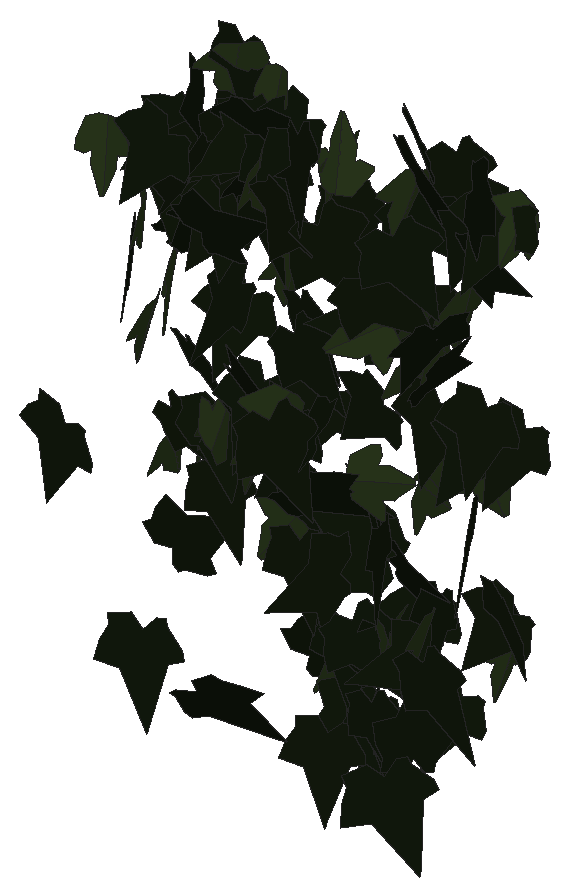
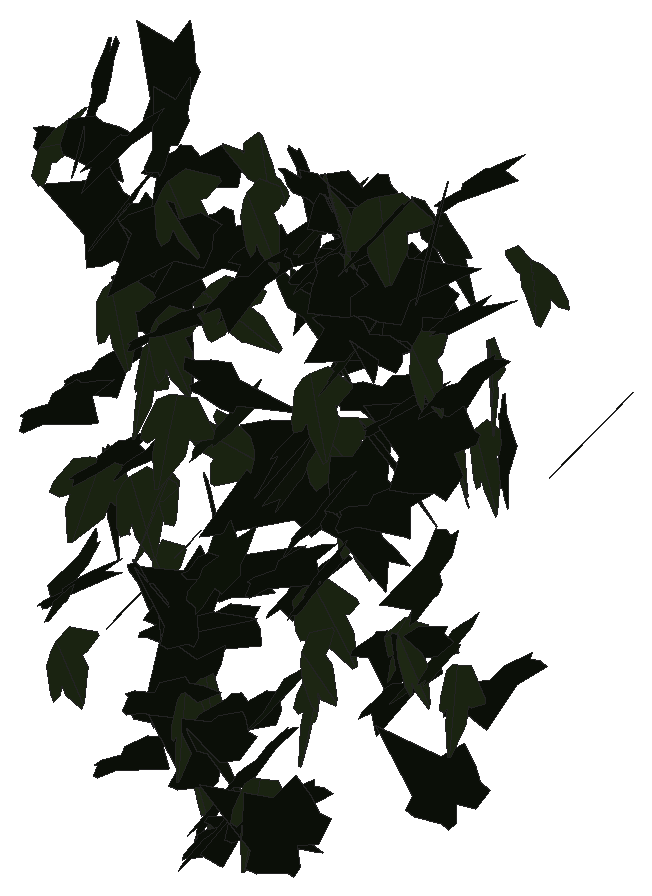
# SketchUp Ruby script. Lengths in inches.
U = 1.inch
M = Sketchup.active_model
def pt(a) = Geom::Point3d.new(a.map { |v| v * U })
def face(e, loops, mat)
  f = e.add_face(loops[0].map { |a| pt(a) })
  loops[1..].each { |l| e.add_face(l.map { |a| pt(a) }).erase! }
  f.material = f.back_material = mat if mat
  f
end
# faces: each face lists its corners as indices into pts; further lists are holes
def faces(e, pts, list, mat = nil) = list.each { |f| face(e, (f[0].is_a?(Array) ? f : [f]).map { |l| l.map { |i| pts[i] } }, mat) }
# xy, xz, yz: faces in a plane at the given z, y or x. An outline is a flat list of corners, or four numbers for a rectangle; further outlines are holes
def ring(l) = l.size == 4 ? [[l[0], l[1]], [l[2], l[1]], [l[2], l[3]], [l[0], l[3]]] : l.each_slice(2).to_a
def flat(e, list, mat, &to3) = list.each { |f| face(e, (f[0].is_a?(Array) ? f : [f]).map { |l| ring(l).map { |u, v| to3.(u, v) } }, mat) }
def xy(e, z, list, mat = nil) = flat(e, list, mat) { |x, y| [x, y, z] }
def xz(e, y, list, mat = nil) = flat(e, list, mat) { |x, z| [x, y, z] }
def yz(e, x, list, mat = nil) = flat(e, list, mat) { |y, z| [x, y, z] }
def lines(e, pts, list) = list.each { |a, b| e.add_line(pt(pts[a]), pt(pts[b])) }
# prism: a flat outline (further loops are holes) pulled along v
def prism(e, loops, v, mat = nil)
  f = face(e, loops, mat); d = Geom::Vector3d.new(v.map { |x| x * U })
  f.pushpull(f.normal.samedirection?(d) ? d.length : -d.length)
end
def box(e, o, s, mat = nil) = prism(e, [[o, [o[0] + s[0], o[1], o[2]], [o[0] + s[0], o[1] + s[1], o[2]], [o[0], o[1] + s[1], o[2]]]], [0, 0, s[2]], mat)
def at(x, y, z, deg = 0) = Geom::Transformation.translation(pt([x, y, z])) * Geom::Transformation.rotation(ORIGIN, Z_AXIS, deg.degrees)
def axes(o, x, y, z) = Geom::Transformation.new([*x, 0, *y, 0, *z, 0, *pt(o).to_a, 1])
def part(name) = M.definitions.add(name)
# library, detail: a bought-in or finely detailed component or shape, given as its bounding box
def library(name, o, s) = part(name).tap { |d| box(d.entities, o, s) }
def detail(e, o, s) = box(e.add_group.entities, o, s)
def put(e, d, t, mat = nil) = e.add_instance(d, t).tap { |i| i.material = mat if mat }
def group(e, t, mat = nil) = e.add_group.tap { |g| g.transformation = t; g.material = mat if mat }.entities
root = M.entities
M.materials.add("efeu1").color = [18, 25, 13]
M.materials.add("efeu2").color = [43, 57, 29]
c1 = part("ivyleaf_9")
p = [[1.54,2.16,1.25],[1.36,2.04,1.19],[-0.21,0.99,0.68],[-0.71,1.11,0.82],[-0.85,0.86,0.67],[-0.8,0.17,0.21],
  [-0.9,-0.01,0.1],[-0.67,-0.16,-0.02],[-0.08,-0.08,-0.05],[-0.03,-0.6,-0.4],[0.65,-0.88,-0.66],[0.83,-0.6,-0.49],
  [1.29,-0.42,-0.43],[1.8125,-0.07,-0.26],[1.21,0.44,0.15]]
faces(c1.entities,p,[[0,1,2,3,4,5,6,7,8,9,10,11,12,13,14]],"efeu1")
c2 = part("ivyleaf_10")
p = [[0,0.5,-0.03],[-0.0625,2.02,-0.43],[-0.19,2.01,-0.46],[-0.54,1.05,-0.29],[-0.52,0.625,-0.18],[-0.83,0.76,-0.28],
  [-1.16,0.64,-0.33],[-1.15,0.33,-0.24],[-0.77,-0.39,0.02],[-0.3,-0.51,0.16],[0.04,-0.48,0.23],[-0.02,2.01,-0.4375],
  [-0.06,2.01,-0.43],[0.04,-0.49,0.23],[0.67,-0.49,0.14],[1.38,0.36,-0.2],[1.375,0.51,-0.24],[0.81,0.65,-0.19],
  [0.62,0.59,-0.15],[0.6,1.09,-0.28],[0.5,1.23,-0.31]]
faces(c2.entities,p,[[0,1,2,3,4,5,6,7,8,9,10],[11,12,0,13,14,15,16,17,18,19,20]],"efeu2")
put(root,c1,axes([577.89,105.38,287.08],[1.36278,0.54862,0.30222],[0.27821,0.11819,-1.46906],[-0.56118,1.39088,0.00562]))
put(root,c1,axes([563.9,114.26,290.22],[-0.08091,-1.18047,0.66258],[0.11331,-0.66733,-1.17511],[1.34895,-0.01475,0.13845]))
put(root,c1,axes([574.375,114.15,293.99],[0.26304,-1.18109,-0.79581],[-0.14529,0.7828,-1.20979],[1.41675,0.29956,0.02369]))
put(root,c1,axes([566.35,116.12,281.01],[-0.09475,-1.31976,-0.20399],[0.02309,0.20285,-1.32313],[1.33524,-0.09716,0.00841]))
put(root,c1,axes([578.76,115.81,278.92],[-0.22824,-1.01787,-0.89838],[0.1809,0.88006,-1.04307],[1.34552,-0.29098,-0.01215]))
put(root,c1,axes([575.25,115.64,293.05],[-0.94436,1.02445,0.23829],[-0.18259,0.15571,-1.39303],[-1.03583,-0.96143,0.0283]))
put(root,c1,axes([575.72,116.52,286.74],[-1.25986,0.4566,0.27428],[-0.252,0.10961,-1.33995],[-0.46927,-1.28471,-0.01684]))
put(root,c1,axes([565.27,118.89,301.64],[-0.52851,-1.00941,0.55527],[-0.07084,-0.58128,-1.12412],[1.14988,-0.49976,0.18595]))
put(root,c1,axes([578.23,118.9375,282.4],[0.70807,-1.23112,-0.31612],[-0.01276,0.35496,-1.41095],[1.27099,0.68942,0.16195]))
put(root,c1,axes([572.15,118.625,288.33],[1.21039,0.63768,0.61607],[0.52332,0.32779,-1.36745],[-0.71576,1.31801,0.04201]))
put(root,c2,axes([569.98,120.21,290.71],[-0.43783,-0.87738,0.74683],[-0.04292,-0.78596,-0.94851],[1.15139,-0.36293,0.24863]))
put(root,c2,axes([561.52,119.76,300.16],[1.20036,-0.19085,0.29262],[0.28978,-0.04099,-1.21543],[0.19514,1.23483,0.00488]))
put(root,c1,axes([571.11,120.01,284.96],[0.15727,-1.22297,-0.12797],[0.00639,0.12983,-1.23283],[1.22963,0.15574,0.02278]))
put(root,c1,axes([566.16,119.18,300.13],[-0.65049,1.03551,0.3217],[-0.19726,0.25588,-1.22251],[-1.06624,-0.67909,0.0299]))
put(root,c1,axes([570.03,120.67,299.14],[-0.21173,-0.90489,0.90272],[0.23072,-0.92705,-0.87516],[1.25718,0.01773,0.31264]))
put(root,c2,axes([577.16,120.29,283.33],[0.4807,-1.10236,0.33779],[0.12234,-0.31513,-1.20254],[1.14644,0.49584,-0.01331]))
put(root,c2,axes([563.58,120.07,292.78],[0.34272,-1.17563,0.02611],[0.00411,-0.026,-1.22456],[1.17591,0.34273,-0.00333]))
put(root,c1,axes([576.95,120.68,281.52],[-0.79447,-0.34135,0.79792],[-0.63668,-0.50589,-0.85035],[0.58977,-1.00595,0.15688]))
put(root,c1,axes([577.22,119.47,277.95],[-0.59743,-0.67037,1.00603],[0.67993,0.74154,0.8979],[-0.9996,0.90506,0.00949]))
put(root,c1,axes([574.73,120.51,286.51],[-0.54702,0.00334,-1.18883],[1.17206,-0.21759,-0.53992],[-0.19905,-1.29043,0.08796]))
put(root,c1,axes([566.18,120.21,297.12],[0.157,-0.2934,1.28344],[1.16543,-0.57029,-0.27293],[0.61243,1.16045,0.19036]))
put(root,c2,axes([574.18,120.09,288.9],[0.25921,-0.06776,-1.21929],[1.20348,-0.19721,0.2668],[-0.2071,-1.23084,0.02437]))
put(root,c1,axes([578.26,119.09,295.24],[0.27353,0.98132,0.76722],[0.21056,0.73777,-1.01872],[-1.22771,0.34517,-0.00378]))
put(root,c1,axes([571.91,120.73,276.32],[-0.22673,-1.19319,-0.1831],[0.02861,0.18094,-1.21453],[1.20682,-0.22846,-0.00561]))
put(root,c2,axes([568.76,120.55,288.57],[0.1236,-1.20506,0.1788],[-0.00327,-0.18005,-1.21119],[1.21825,0.12178,-0.02139]))
put(root,c2,axes([575.41,120.62,276.25],[0.58962,-1.08793,0.02339],[0.01036,-0.02099,-1.23743],[1.08813,0.58971,-0.00089]))
put(root,c1,axes([575.9,121.23,302.59],[0.30446,-0.52323,1.26611],[0.66648,-1.07659,-0.60518],[1.19691,0.73257,0.01492]))
put(root,c1,axes([575.5,120.46,299.88],[-0.04129,-0.87034,-0.91332],[0.14047,0.90496,-0.86872],[1.25376,-0.13005,0.06725]))
put(root,c1,axes([567.95,121.35,289.66],[0.97732,-0.73267,0.40156],[-0.30722,0.25954,1.22125],[-0.77696,-1.02423,0.02221]))
put(root,c2,axes([574.05,121.05,295.14],[0.72605,0.11446,-1.00994],[-1.01361,-0.01047,-0.72987],[-0.07534,1.2438,0.0868]))
put(root,c2,axes([562.6,120.77,296.79],[0.58017,-1.01804,-0.39809],[-0.05093,0.42503,-1.16114],[1.09192,0.56074,0.15736]))
put(root,c2,axes([569.86,121.02,284.99],[-0.93809,-0.08041,0.78306],[-0.74688,-0.29386,-0.92492],[0.24864,-1.1861,0.17606]))
put(root,c1,axes([574.13,120.39,297.6],[0.18492,-0.51713,-1.20247],[0.04793,1.21627,-0.5157],[1.30808,0.02854,0.18889]))
put(root,c1,axes([561.35,121.77,294.41],[-0.17003,-0.1695,-1.27422],[1.18432,-0.52035,-0.08882],[-0.49974,-1.17549,0.22305]))
put(root,c1,axes([569.14,122.0625,289.07],[0.03941,-1.2902,0.50679],[-0.02468,-0.50757,-1.29026],[1.38595,0.02765,-0.03738]))
put(root,c1,axes([573.95,121.61,284.69],[-0.79672,-0.92263,-0.46111],[-0.30433,-0.34644,1.21901],[-0.98552,0.85286,-0.00366]))
put(root,c1,axes([569.55,121.77,301.7],[-0.64683,-0.14753,-1.1372],[1.14315,0.0202,-0.65283],[0.0906,-1.30813,0.11817]))
put(root,c1,axes([576.59,121.74,283.55],[-0.8172,-0.09349,-0.84368],[0.84407,0.03448,-0.8214],[0.08986,-1.17406,0.04306]))
put(root,c1,axes([571.26,121.125,298.59],[0.32352,-0.9443,-1.00575],[-0.11667,1.01061,-0.98639],[1.37464,0.30801,0.15299]))
put(root,c1,axes([573.16,122.51,290.77],[-0.51599,-0.70657,0.92485],[0.10306,-1.03544,-0.73355],[1.1593,-0.22244,0.47686]))
put(root,c2,axes([562.93,122.15,293.5],[0.64905,-0.79377,0.75091],[0.56877,-0.50031,-1.02049],[0.93297,0.85721,0.09973]))
put(root,c1,axes([567.26,122.55,300.82],[-0.82698,-0.61661,0.73916],[-0.44091,-0.6236,-1.0135],[0.85567,-0.91726,0.19214]))
put(root,c2,axes([567.83,121.46,299.97],[0.27421,-1.14773,-0.41918],[0.07985,0.44552,-1.16761],[1.21927,0.22895,0.17074]))
put(root,c2,axes([571.76,121.6,300.89],[1.22195,-0.11879,0.25277],[-0.23605,0.16708,1.21964],[-0.14928,-1.23659,0.14051]))
put(root,c1,axes([578.87,121.18,302.86],[0.53115,-0.29829,-1.28915],[-1.07354,0.71496,-0.60774],[0.77356,1.19702,0.04175]))
put(root,c1,axes([568.79,122.93,286.5625],[-0.3129,-0.66714,1.03647],[-0.18543,-1.0317,-0.72004],[1.21859,-0.32829,0.15657]))
put(root,c1,axes([576.28,121.83,295.47],[-0.13088,1.13232,-0.66665],[0.05253,-0.6649,-1.13966],[-1.31293,-0.13948,0.02086]))
put(root,c1,axes([577.69,122.58,287.45],[-0.60065,0.20524,-1.24958],[1.16112,-0.46265,-0.63412],[-0.50534,-1.30698,0.02824]))
put(root,c1,axes([563.8,122.97,300.64],[-0.04151,-0.17225,1.30547],[-0.05253,-1.30486,-0.17384],[1.31574,-0.05753,0.03424]))
put(root,c1,axes([569.25,122.51,302.11],[-1.19732,-0.19335,-0.15528],[0.1564,0.00537,-1.21267],[0.19244,-1.20733,0.01947]))
put(root,c1,axes([567.32,121.84,302.04],[0.71611,0.6531,-0.8491],[-0.65285,-0.54368,-0.96878],[-0.8493,0.96861,0.02874]))
put(root,c1,axes([567.82,122.6,300.03],[0.25555,-1.32619,-0.01949],[-0.00444,0.019,-1.35059],[1.32633,0.25559,-0.00076]))
put(root,c1,axes([572.13,122.79,276.66],[-1.05614,-0.45578,0.43483],[-0.39983,-0.17091,-1.15029],[0.48677,-1.12929,-0.00141]))
put(root,c1,axes([574,122.54,283.78],[0.49409,-0.48091,1.03658],[0.77627,-0.68748,-0.68896],[0.83855,0.91977,0.02702]))
put(root,c1,axes([567.09,122.66,289.51],[-1.06388,-0.42242,-0.52722],[0.51245,0.13628,-1.14326],[0.44022,-1.1795,0.05673]))
put(root,c1,axes([579.05,123.19,283.18],[-0.57956,-0.86263,0.60045],[-0.06256,-0.65616,-1.00304],[1.04916,-0.51564,0.27188]))
put(root,c1,axes([569.26,122.11,292.65],[0.61896,-0.95162,-0.6698],[-0.22478,0.64659,-1.12638],[1.14179,0.64317,0.14135]))
put(root,c1,axes([572.67,122.59,277.15],[0.39567,-1.07385,-0.1602],[-0.0226,0.16232,-1.14391],[1.0855,0.3948,0.03458]))
put(root,c1,axes([577.96,123.04,291.99],[-0.32568,-1.20389,0.10958],[-0.00008,-0.11346,-1.24681],[1.20886,-0.32435,0.02944]))
put(root,c2,axes([573.96,122.01,280.39],[-0.86404,0.37667,0.68619],[-0.65681,0.20714,-0.94075],[-0.42584,-1.08376,0.05869]))
put(root,c1,axes([562.76,123.39,299.03],[-0.68353,-0.64737,0.81932],[-0.28756,-0.82468,-0.89151],[1.00384,-0.67705,0.3025]))
put(root,c1,axes([572.6,122.84,276.11],[-0.09063,-1.14355,-0.11002],[-0.01146,0.11126,-1.14696],[1.14877,-0.08911,-0.02012]))
put(root,c1,axes([572.07,122.21,280.78],[0.1626,-0.85196,-0.84036],[0.04388,0.85176,-0.85502],[1.19587,0.08459,0.14563]))
put(root,c1,axes([572.43,123.39,285.82],[-0.23204,-0.6704,1.11977],[0.42225,-1.11472,-0.57988],[1.23492,0.25519,0.40868]))
put(root,c1,axes([578.73,123.09,283.71],[0.53554,-1.02212,0.40608],[0.15559,-0.37671,-1.15339],[1.08877,0.55659,-0.03491]))
put(root,c1,axes([565.77,122.9,293.35],[-1.23523,0.22734,-0.40711],[0.39898,-0.08129,-1.25595],[-0.24132,-1.29805,0.00736]))
put(root,c1,axes([570.83,123.17,279.5],[0.18261,-1.20725,0.10411],[0.01842,-0.10251,-1.22098],[1.21159,0.18352,0.00287]))
put(root,c1,axes([564.71,122.93,284.45],[0.18753,-1.14588,-0.32734],[0.00398,0.33197,-1.15981],[1.19172,0.17921,0.05539]))
put(root,c1,axes([565.46,123.5625,299.9375],[-0.31332,-0.64155,-1.03911],[-0.12434,-1.05043,0.68603],[-1.21485,0.27296,0.19778]))
put(root,c1,axes([578.79,123.36,301.08],[-0.98853,-0.81503,-0.06027],[0.04514,0.04,-1.28119],[0.81601,-0.98955,-0.00215]))
put(root,c1,axes([567.14,122.53,299.29],[-0.08221,1.21274,-0.3604],[0.01764,-0.36002,-1.21551],[-1.26504,-0.08383,0.00648]))
put(root,c1,axes([573.74,122.81,279.9],[-0.85773,0.78078,-0.06225],[0.03978,-0.04876,-1.15984],[-0.78225,-0.8586,0.00927]))
put(root,c1,axes([562.63,122.84,280.66],[-0.07925,0.05703,1.23905],[1.14165,-0.48202,0.09521],[0.4849,1.14419,-0.02165]))
put(root,c1,axes([569.27,123.75,282.75],[0.05959,-1.11553,0.60498],[0.20415,-0.58933,-1.10679],[1.25249,0.14914,0.15162]))
put(root,c1,axes([574.15,123.73,302.42],[0.23642,-0.65477,1.04571],[0.39283,-0.96938,-0.69579],[1.16958,0.45794,0.02231]))
put(root,c1,axes([576.07,123.74,278.11],[-0.55613,-0.98352,0.2666],[-0.0364,-0.28436,-1.12494],[1.01836,-0.54726,0.10538]))
put(root,c2,axes([575.3,122.39,287.94],[0.35288,-0.86341,-0.86324],[0.21265,0.9283,-0.84156],[1.20226,0.08923,0.40222]))
put(root,c2,axes([574.58,123.39,294.68],[0.17718,-1.18072,0.34133],[0.02181,-0.34179,-1.19362],[1.22888,0.1763,-0.02803]))
put(root,c1,axes([562.56,122.82,286.68],[0.87331,-0.76684,-0.3514],[-0.0934,0.41478,-1.13728],[0.83833,0.84504,0.23935]))
put(root,c1,axes([566.3125,123.54,297.08],[0.5217,-1.14333,0.15498],[0.0618,-0.14215,-1.25673],[1.15213,0.52534,-0.00276]))
put(root,c1,axes([562.96,123.29,289.51],[0.92191,-0.84276,0.21842],[0.15633,-0.1527,-1.24904],[0.85645,0.93504,-0.00712]))
put(root,c2,axes([570.63,123.47,300.98],[0.26889,-1.18359,0.29569],[0.05014,-0.29181,-1.21366],[1.21894,0.2731,-0.01531]))
put(root,c1,axes([572.27,123.64,276.42],[0.2318,-1.16401,0.1185],[0.02964,-0.11492,-1.18685],[1.16965,0.2336,0.00659]))
put(root,c2,axes([579.04,124.05,300.61],[-0.39437,-0.50394,1.0881],[0.54717,-1.09486,-0.30875],[1.06701,0.37519,0.5605]))
put(root,c1,axes([561.63,123.72,297.52],[-0.0306,-1.24024,-0.05442],[0.00363,0.05435,-1.24062],[1.24143,-0.03073,0.00229]))
put(root,c1,axes([576.87,123.29,298.37],[0.60096,0.01997,-1.10127],[1.04017,0.40232,0.57492],[0.36226,-1.18831,0.17613]))
put(root,c2,axes([562.28,122.99,285.36],[0.08574,-1.08727,-0.50464],[0.02221,0.50728,-1.08919],[1.19847,0.06838,0.05628]))
put(root,c2,axes([573.82,123.73,300.41],[-0.13628,-1.16164,0.45441],[0.07742,-0.46411,-1.16321],[1.24495,-0.0983,0.12208]))
put(root,c1,axes([574.73,124.12,290.56],[-0.17607,-1.20745,0.37751],[0.05421,-0.388,-1.21571],[1.26392,-0.15156,0.10473]))
put(root,c2,axes([567.02,123.59,302.6],[1.04102,-0.56831,0.28773],[0.24019,-0.16037,-1.18579],[0.58998,1.06808,-0.02495]))
put(root,c1,axes([578.86,124.18,290.87],[-0.53124,-1.08065,0.28391],[-0.10299,-0.26567,-1.20392],[1.11256,-0.54059,0.02412]))
put(root,c1,axes([564.0625,124.31,295.73],[-0.50955,-0.97476,0.52143],[-0.0376,-0.55854,-1.08088],[1.10482,-0.46858,0.2037]))
put(root,c1,axes([575.98,124.34,299.2],[0.00271,-1.0552,0.65451],[0.02732,-0.6543,-1.05497],[1.2414,0.01671,0.02179]))
put(root,c1,axes([572.6,123.72,293.73],[-0.88933,0.12566,0.81012],[-0.81109,0.03894,-0.89644],[-0.11921,-1.20237,0.05563]))
put(root,c2,axes([564.76,122.5625,286.34],[0.15334,0.52626,-1.12057],[-0.11136,1.13041,0.51564],[1.23297,0.03665,0.18593]))
put(root,c1,axes([574.08,124.41,295.53],[-0.52362,-1.02596,0.45091],[0.02708,-0.50914,-1.12701],[1.12035,-0.4672,0.23799]))
put(root,c2,axes([568.43,123.11,282.95],[-0.92891,0.77239,0.36964],[-0.27685,0.24518,-1.20803],[-0.8103,-0.96923,-0.01101]))
put(root,c2,axes([563.73,123.92,286.61],[0.48002,-1.0968,0.32795],[0.09795,-0.31496,-1.19672],[1.14058,0.48864,-0.03524]))
put(root,c1,axes([564.03,123.78,286.82],[-0.34826,-1.04427,-0.57352],[0.26951,0.51298,-1.09769],[1.16052,-0.43251,0.08282]))
put(root,c1,axes([576.55,124.5,289.59],[-0.5061,-0.9947,0.53894],[-0.10536,-0.5464,-1.10741],[1.12641,-0.49803,0.13856]))
put(root,c1,axes([570.57,123.86,298.53],[0.13608,-1.1957,-0.33329],[-0.05078,0.32964,-1.20335],[1.24024,0.14469,-0.01271]))
put(root,c2,axes([578.42,124.08,281.27],[0.05087,-1.07595,0.45158],[0.17304,-0.44006,-1.06799],[1.15397,0.11342,0.14024]))
put(root,c1,axes([564.98,124.32,291.875],[-0.59813,-1.04604,0.07859],[-0.02907,-0.0739,-1.20492],[1.04859,-0.59872,0.01143]))
put(root,c1,axes([562.42,123.27,294.42],[0.80537,0.85603,-0.56737],[0.39586,0.40655,1.1753],[0.94762,-0.89736,-0.00877]))
put(root,c1,axes([572.63,123.02,278.79],[-0.2359,-0.15567,1.19531],[1.01108,0.63758,0.28258],[-0.65629,1.03822,0.00569]))
put(root,c2,axes([567.78,123.83,295.06],[-0.13105,-1.21928,0.03461],[-0.0031,-0.03448,-1.22631],[1.21977,-0.13109,0.0006]))
put(root,c1,axes([565.64,123.72,298],[-0.01264,-0.70865,-1.00065],[0.77622,0.77004,-0.55514],[0.94919,-0.63915,0.44064]))
put(root,c2,axes([575.36,123.96,288.53],[-0.08342,-1.17276,0.1863],[-0.01723,-0.18554,-1.17571],[1.18734,-0.08509,-0.00397]))
put(root,c1,axes([574.19,124.33,281.38],[-0.76306,-0.8808,-0.0431],[0.02913,0.03178,-1.16536],[0.88137,-0.76361,0.00121]))
put(root,c2,axes([570.49,123.47,278.28],[-0.14492,-1.12045,-0.49738],[0.13127,0.48378,-1.12806],[1.21884,-0.18533,0.06236]))
put(root,c2,axes([564.85,123.91,302.96],[-0.68573,-0.99875,0.1184],[-0.03671,-0.11835,-1.21095],[1.00507,-0.68574,0.03655]))
put(root,c1,axes([564.47,124.24,296.53],[-0.66865,-0.97782,-0.33325],[0.15068,0.3004,-1.18378],[1.022,-0.68403,-0.0435]))
put(root,c1,axes([575.8,123.98,302.18],[0.41022,-1.1087,-0.42821],[-0.00432,0.45161,-1.17341],[1.18851,0.38431,0.14354]))
put(root,c2,axes([576.07,124.22,295.84],[0.00443,-1.23945,0.07256],[0.02395,-0.07247,-1.23923],[1.24134,0.00582,0.02365]))
put(root,c1,axes([568.61,123.96,277.42],[0.25227,-0.09617,1.25178],[1.22073,-0.2795,-0.26749],[0.2933,1.24599,0.03662]))
put(root,c2,axes([562.6,124.58,298.4],[0.38291,-1.08925,0.4376],[0.16985,-0.40404,-1.15433],[1.16151,0.41817,0.02453]))
put(root,c2,axes([567.1875,124.76,285.22],[0.39538,-0.93989,0.65121],[0.26274,-0.59593,-1.01963],[1.11285,0.47463,0.00936]))
put(root,c2,axes([577.13,124.01,288.61],[-0.80103,-0.79664,-0.36954],[0.3184,0.20268,-1.12711],[0.81842,-0.85857,0.07681]))
put(root,c1,axes([568.45,125.01,288.49],[-0.46888,-1.07306,0.3067],[-0.07553,-0.3014,-1.16997],[1.11347,-0.4723,0.04979]))
put(root,c2,axes([573.74,123.95,292.16],[-0.34235,-1.11856,-0.45271],[0.17538,0.41946,-1.16902],[1.19389,-0.38236,0.04191]))
put(root,c1,axes([567.72,124.43,292.56],[0.7304,-0.95556,-0.00697],[-0.01188,-0.0003,-1.20269],[0.95551,0.73043,-0.00962]))
put(root,c2,axes([573.21,124,280.91],[0.18736,-1.05396,-0.44715],[0.05547,0.46092,-1.06318],[1.14354,0.15032,0.12484]))
put(root,c1,axes([573.81,123.78,299.48],[-0.04073,-0.52572,-1.14109],[0.14192,1.13246,-0.52681],[1.24833,-0.1459,0.02266]))
put(root,c2,axes([574.91,123.88,293.66],[0.25091,-1.03158,-0.63435],[0.06374,0.65817,-1.04512],[1.20934,0.17934,0.1867]))
put(root,c1,axes([564.4,124.88,302.73],[0.19316,-1.19003,0.23852],[0.03293,-0.23629,-1.20559],[1.21325,0.19587,-0.00525]))
